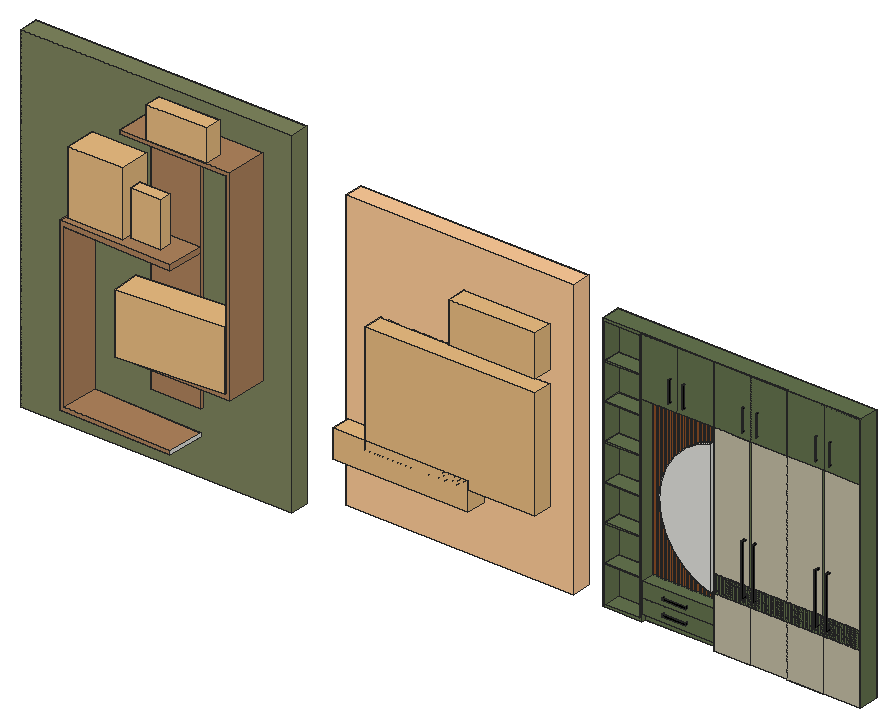
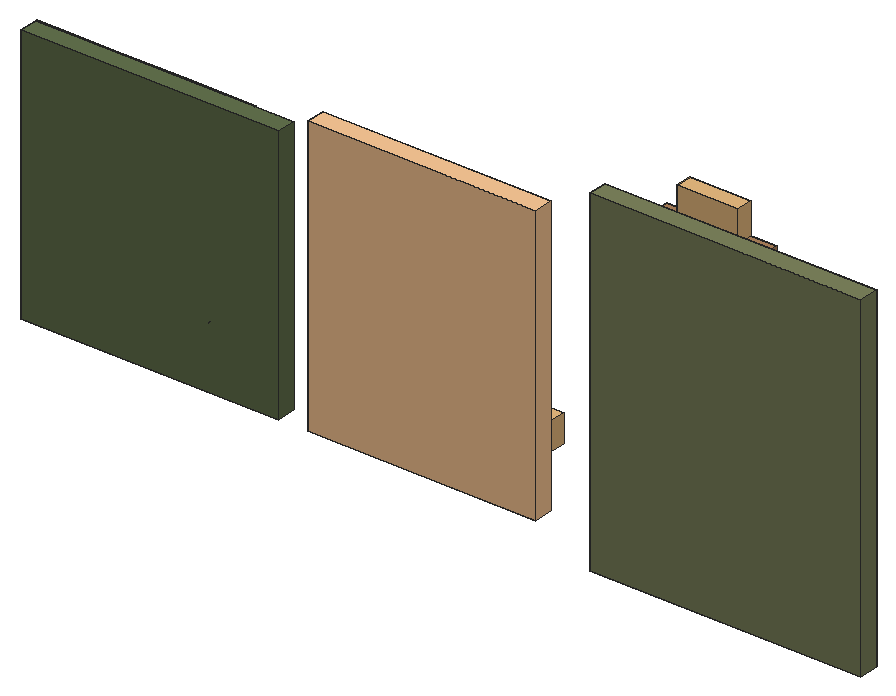
# SketchUp Ruby script. Lengths in inches.
U = 1.inch
M = Sketchup.active_model
def pt(a) = Geom::Point3d.new(a.map { |v| v * U })
def face(e, loops, mat)
  f = e.add_face(loops[0].map { |a| pt(a) })
  loops[1..].each { |l| e.add_face(l.map { |a| pt(a) }).erase! }
  f.material = f.back_material = mat if mat
  f
end
# faces: each face lists its corners as indices into pts; further lists are holes
def faces(e, pts, list, mat = nil) = list.each { |f| face(e, (f[0].is_a?(Array) ? f : [f]).map { |l| l.map { |i| pts[i] } }, mat) }
# xy, xz, yz: faces in a plane at the given z, y or x. An outline is a flat list of corners, or four numbers for a rectangle; further outlines are holes
def ring(l) = l.size == 4 ? [[l[0], l[1]], [l[2], l[1]], [l[2], l[3]], [l[0], l[3]]] : l.each_slice(2).to_a
def flat(e, list, mat, &to3) = list.each { |f| face(e, (f[0].is_a?(Array) ? f : [f]).map { |l| ring(l).map { |u, v| to3.(u, v) } }, mat) }
def xy(e, z, list, mat = nil) = flat(e, list, mat) { |x, y| [x, y, z] }
def xz(e, y, list, mat = nil) = flat(e, list, mat) { |x, z| [x, y, z] }
def yz(e, x, list, mat = nil) = flat(e, list, mat) { |y, z| [x, y, z] }
def lines(e, pts, list) = list.each { |a, b| e.add_line(pt(pts[a]), pt(pts[b])) }
# prism: a flat outline (further loops are holes) pulled along v
def prism(e, loops, v, mat = nil)
  f = face(e, loops, mat); d = Geom::Vector3d.new(v.map { |x| x * U })
  f.pushpull(f.normal.samedirection?(d) ? d.length : -d.length)
end
def box(e, o, s, mat = nil) = prism(e, [[o, [o[0] + s[0], o[1], o[2]], [o[0] + s[0], o[1] + s[1], o[2]], [o[0], o[1] + s[1], o[2]]]], [0, 0, s[2]], mat)
def at(x, y, z, deg = 0) = Geom::Transformation.translation(pt([x, y, z])) * Geom::Transformation.rotation(ORIGIN, Z_AXIS, deg.degrees)
def axes(o, x, y, z) = Geom::Transformation.new([*x, 0, *y, 0, *z, 0, *pt(o).to_a, 1])
def part(name) = M.definitions.add(name)
# library, detail: a bought-in or finely detailed component or shape, given as its bounding box
def library(name, o, s) = part(name).tap { |d| box(d.entities, o, s) }
def detail(e, o, s) = box(e.add_group.entities, o, s)
def put(e, d, t, mat = nil) = e.add_instance(d, t).tap { |i| i.material = mat if mat }
def group(e, t, mat = nil) = e.add_group.tap { |g| g.transformation = t; g.material = mat if mat }.entities
root = M.entities
M.materials.add("[Color A01]").color = [101, 116, 79]
M.materials.add("[Color A01]1").color = [196, 189, 165]
M.materials.add("[Color A01]2").color = [176, 132, 93]
M.materials.add("[Color A02]").color = [127, 133, 94]
M.materials.add("[Color C02]").color = [255, 204, 153]
M.materials.add("[Color M09]").color = [0, 0, 0]
M.materials.add("[Wood Cherry Original]").color = [152, 86, 42]
c1 = library("Untitled",[0,0,0],[7.78,10.125,9.38])
c2 = library("Ceramic Birds on",[-120.01,56.07,-27.09],[117.74,27.05,54.18])
c3 = library("SimLab\#1",[-237.64,52,0],[43.92,43.98,50.37])
c4 = part("Vertical wood slat")
box(c4.entities,[0,-2,0],[1,2,76],"[Wood Cherry Original]")
c5 = part("Group\#7")
prism(c5.entities,[[[0.625,2,0],[0.625,2,0.59],[0.625,0.59,0.59],[0.625,0.59,23.53],[0.625,2,23.53],[0.625,2,24.13],[0.625,0,24.13],[0.625,0,0]]],[-0.625,0,0])
c6 = part("Group\#5")
prism(c6.entities,[[[0.5,1,9.71],[0.5,1,10],[0.5,0,10],[0.5,0,0],[0.5,1,0],[0.5,1,0.29],[0.5,0.29,0.29],[0.5,0.29,9.71]]],[-0.5,0,0])
c7 = library("Group\#37",[208.35,-82.82,84.7],[13.92,5.45,20.99])
xy(root,5.8,[[84.22,0.51,32.41,1.51,32.74,19,84.56,18]],"[Color A01]2")
xy(root,84.7,[[84.22,0.51,84.56,18,32.74,19,32.41,1.51]],"[Color A01]2")
p = [[84.22,0.51,5.8],[84.22,0.51,7.18],[34.4,1.47,7.8],[34.4,1.47,82.7],[84.22,0.51,82.08],[84.22,0.51,84.7],
  [32.41,1.51,84.7],[32.41,1.51,5.8],[84.56,18,5.8],[84.56,18,7.18],[32.74,19,84.7],[32.74,19,5.8],
  [84.56,18,84.7],[84.56,18,82.08],[34.74,18.96,82.7],[34.74,18.96,7.8]]
faces(root,p,[[0,1,2,3,4,5,6,7],[10,11,7,6],[3,2,15,14],[4,3,14,13],[4,13,12,5]],"[Color A01]2")
faces(root,p,[[8,9,1,0],[12,13,14,15,9,8,11,10]])
put(root,c1,axes([110.34,0.03,40.32],[-0.12671,1.68524,0],[-4.76654,-0.3584,0],[0,0,3]))
put(root,c2,axes([102.2,-15.7,140.64],[0.23902,0,0],[0,0.28,0],[0,0,0.2698]))
put(root,c3,axes([171.33,-17.61,84.65],[0.58,0,0],[0,0.4272,0],[0,0,0.59]))
g1 = group(root,at(270.37,16.53,0))
prism(g1,[[[39.05,2.47,12.84],[39.35,2.47,12.84],[39.35,1.47,12.84],[28.35,1.47,12.84],[28.35,2.47,12.84],[28.65,2.47,12.84],[28.65,1.77,12.84],[39.05,1.77,12.84]]],[0,0,1],"[Color M09]")
prism(g1,[[[39.05,2.47,6],[39.35,2.47,6],[39.35,1.47,6],[28.35,1.47,6],[28.35,2.47,6],[28.65,2.47,6],[28.65,1.77,6],[39.05,1.77,6]]],[0,0,1],"[Color M09]")
put(g1,c4,at(34.23,10.47,17))
put(g1,c4,at(24.23,10.47,17))
put(g1,c4,at(46.23,10.47,17))
put(g1,c4,at(48.23,10.47,17))
put(g1,c4,at(44.23,10.47,17))
put(g1,c4,at(18.23,10.47,17))
put(g1,c4,at(20.23,10.47,17))
put(g1,c4,at(26.23,10.47,17))
put(g1,c4,at(42.23,10.47,17))
put(g1,c4,at(28.23,10.47,17))
put(g1,c4,at(36.23,10.47,17))
put(g1,c4,at(30.23,10.47,17))
put(g1,c4,at(22.23,10.47,17))
put(g1,c4,at(32.23,10.47,17))
put(g1,c4,at(38.23,10.47,17))
put(g1,c4,at(40.23,10.47,17))
put(g1,c4,at(50.23,10.47,17))
put(g1,c4,at(54.23,10.47,17))
put(g1,c4,at(58.23,10.47,17))
put(g1,c4,at(52.23,10.47,17))
put(g1,c4,at(56.23,10.47,17))
g2 = group(g1,at(23.23,8.39,20.33))
xz(g2,0,[[[24,0,17.44,2.49,11.58,6.35,6.7,11.4,3.04,17.38,0.77,24.02,0,31,0.77,37.98,3.04,44.62,6.7,50.6,11.58,55.65,17.44,59.51,24,62],[21.5,3.63,21.5,58.37,18.59,57.27,13.1875,53.71,8.69,49.06,5.32,43.54,3.23,37.43,2.52,31,3.23,24.57,5.32,18.46,8.69,12.94,13.1875,8.29,18.59,4.73]]])
g3 = group(g1,at(23.23,6.31,20.33))
xz(g3,0,[[24,0,24,62,17.44,59.51,11.58,55.65,6.7,50.6,3.04,44.62,0.77,37.98,0,31,0.77,24.02,3.04,17.38,6.7,11.4,11.58,6.35,17.44,2.49]])
xz(g3,2,[[[24,0,17.44,2.49,11.58,6.35,6.7,11.4,3.04,17.38,0.77,24.02,0,31,0.77,37.98,3.04,44.62,6.7,50.6,11.58,55.65,17.44,59.51,24,62],[21.5,3.63,21.5,58.37,18.59,57.27,13.1875,53.71,8.69,49.06,5.32,43.54,3.23,37.43,2.52,31,3.23,24.57,5.32,18.46,8.69,12.94,13.1875,8.29,18.59,4.73]],[21.5,3.63,18.59,4.73,13.1875,8.29,8.69,12.94,5.32,18.46,3.23,24.57,2.52,31,3.23,37.43,5.32,43.54,8.69,49.06,13.1875,53.71,18.59,57.27,21.5,58.37]])
yz(g3,24,[[0,0,2,62]])
p = [[24,0,0],[17.44,0,2.49],[17.44,2,2.49],[24,2,0],[11.58,0,6.35],[11.58,2,6.35],
  [6.7,0,11.4],[6.7,2,11.4],[3.04,0,17.38],[3.04,2,17.38],[0.77,0,24.02],[0.77,2,24.02],
  [0,0,31],[0,2,31],[0.77,0,37.98],[0.77,2,37.98],[3.04,0,44.62],[3.04,2,44.62],
  [6.7,0,50.6],[6.7,2,50.6],[11.58,0,55.65],[11.58,2,55.65],[17.44,0,59.51],[17.44,2,59.51],
  [24,0,62],[24,2,62]]
faces(g3,p,[[0,1,2,3],[1,4,5,2],[4,6,7,5],[6,8,9,7],[8,10,11,9],[10,12,13,11],[12,14,15,13],[14,16,17,15],
  [16,18,19,17],[18,20,21,19],[20,22,23,21],[22,24,25,23]])
g4 = group(g1,at(0,2.47,0),"[Color A01]")
xy(g4,0,[[52.232,-0.472,69.056,0],[69.295,-0.472,85.998,0],[86.234,-0.472,102.94,0],[103.176,-0.472,119.882,0],[0,0,0,9,120,9,120,0,52.232,0,52.232,8,18.232,8,18.232,0]])
xy(g4,1,[[1,0,17.232,8]])
xy(g4,17.857,[[1,0,17.232,8]])
xy(g4,18.357,[[1,0,17.232,8]])
xy(g4,34.714,[[1,0,17.232,8]])
xy(g4,35.214,[[1,0,17.232,8]])
xy(g4,51.571,[[1,0,17.232,8]])
xy(g4,52.071,[[1,0,17.232,8]])
xy(g4,68.429,[[1,0,17.232,8]])
xy(g4,68.929,[[1,0,17.232,8]])
xy(g4,85.286,[[1,0,17.232,8]])
xy(g4,85.786,[[1,0,17.232,8]])
xy(g4,93,[[18.232,-0.472,52.037,0],[52.232,-0.472,52.273,0],[52.273,-0.472,69.056,0],[69.056,-0.472,69.295,0],[69.295,-0.472,85.959,0],
  [85.959,-0.472,85.998,0],[86.196,-0.472,86.234,0],[86.234,-0.472,102.94,0],[102.94,-0.472,103.176,0],[103.176,-0.472,119.882,0],
  [119.882,-0.472,120,0],[18.232,0,52.037,8],[52.037,0,52.155,8],[52.155,0,52.232,8]])
xy(g4,102.143,[[1,0,17.232,8]])
xy(g4,102.643,[[1,0,17.232,8]])
xy(g4,119,[[1,0,17.232,8]])
xy(g4,120,[[18.232,-0.472,52.037,0],[52.273,-0.472,85.959,0],[86.196,-0.472,120,0],[0,0,120,9]])
xz(g4,-0.472,[[52.81,24,53.232,32],[53.81,24,54.232,32],[54.81,24,55.232,32],[55.81,24,56.232,32],[56.81,24,57.232,32],
  [57.81,24,58.232,32],[58.81,24,59.232,32],[59.81,24,60.232,32],[60.81,24,61.232,32],[61.81,24,62.232,32],
  [62.81,24,63.232,32],[63.81,24,64.232,32],[64.81,24,65.232,32],[65.81,24,66.232,32],[66.81,24,67.232,32],
  [67.81,24,68.232,32],[68.81,24,69.232,32],[69.81,24,70.232,32],[70.81,24,71.232,32],[71.81,24,72.232,32],
  [72.81,24,73.232,32],[73.81,24,74.232,32],[74.81,24,75.232,32],[75.81,24,76.232,32],[76.81,24,77.232,32],
  [77.81,24,78.232,32],[78.81,24,79.232,32],[79.81,24,80.232,32],[80.81,24,81.232,32],[81.81,24,82.232,32],
  [82.81,24,83.232,32],[83.81,24,84.232,32],[84.81,24,85.232,32],[85.81,24,86.232,32],[86.81,24,87.232,32],
  [87.81,24,88.232,32],[88.81,24,89.232,32],[89.81,24,90.232,32],[90.81,24,91.232,32],[91.81,24,92.232,32],
  [92.81,24,93.232,32],[93.81,24,94.232,32],[94.81,24,95.232,32],[95.81,24,96.232,32],[96.81,24,97.232,32],
  [97.81,24,98.232,32],[98.81,24,99.232,32],[99.81,24,100.232,32],[100.81,24,101.232,32],[101.81,24,102.232,32],
  [102.81,24,103.232,32],[103.81,24,104.232,32],[104.81,24,105.232,32],[105.81,24,106.232,32],[106.81,24,107.232,32],
  [107.81,24,108.232,32],[108.81,24,109.232,32],[109.81,24,110.232,32],[110.81,24,111.232,32],[111.81,24,112.232,32],
  [112.81,24,113.232,32],[113.81,24,114.232,32],[114.81,24,115.232,32],[115.81,24,116.232,32],[116.81,24,117.232,32],
  [117.81,24,118.232,32],[118.81,24,119.232,32],[119.81,24,119.882,32],[69.056,32,69.295,93],[102.94,32,103.176,93]])
xz(g4,-0.472,[[52.232,24,52.81,32],[53.232,24,53.81,32],[54.232,24,54.81,32],[55.232,24,55.81,32],[56.232,24,56.81,32],
  [57.232,24,57.81,32],[58.232,24,58.81,32],[59.232,24,59.81,32],[60.232,24,60.81,32],[61.232,24,61.81,32],
  [62.232,24,62.81,32],[63.232,24,63.81,32],[64.232,24,64.81,32],[65.232,24,65.81,32],[66.232,24,66.81,32],
  [67.232,24,67.81,32],[68.232,24,68.81,32],[69.232,24,69.81,32],[70.232,24,70.81,32],[71.232,24,71.81,32],
  [72.232,24,72.81,32],[73.232,24,73.81,32],[74.232,24,74.81,32],[75.232,24,75.81,32],[76.232,24,76.81,32],
  [77.232,24,77.81,32],[78.232,24,78.81,32],[79.232,24,79.81,32],[80.232,24,80.81,32],[81.232,24,81.81,32],
  [82.232,24,82.81,32],[83.232,24,83.81,32],[84.232,24,84.81,32],[85.232,24,85.81,32],[86.232,24,86.81,32],
  [87.232,24,87.81,32],[88.232,24,88.81,32],[89.232,24,89.81,32],[90.232,24,90.81,32],[91.232,24,91.81,32],
  [92.232,24,92.81,32],[93.232,24,93.81,32],[94.232,24,94.81,32],[95.232,24,95.81,32],[96.232,24,96.81,32],
  [97.232,24,97.81,32],[98.232,24,98.81,32],[99.232,24,99.81,32],[100.232,24,100.81,32],[101.232,24,101.81,32],
  [102.232,24,102.81,32],[103.232,24,103.81,32],[104.232,24,104.81,32],[105.232,24,105.81,32],[106.232,24,106.81,32],
  [107.232,24,107.81,32],[108.232,24,108.81,32],[109.232,24,109.81,32],[110.232,24,110.81,32],[111.232,24,111.81,32],
  [112.232,24,112.81,32],[113.232,24,113.81,32],[114.232,24,114.81,32],[115.232,24,115.81,32],[116.232,24,116.81,32],
  [117.232,24,117.81,32],[118.232,24,118.81,32],[119.232,24,119.81,32],[18.232,93,35.135,120],[35.135,93,52.037,120],
  [52.273,93,69.116,120],[69.116,93,85.959,120],[86.196,93,103.098,120],[103.098,93,120,120]],"[Color A01]")
xz(g4,-0.472,[[52.232,0,69.056,24],[69.295,0,85.998,24],[86.234,0,102.94,24],[103.176,0,119.882,24],[52.232,32,69.056,93],
  [69.295,32,85.998,93],[86.234,32,102.94,93],[103.176,32,119.882,93]],"[Color A01]1")
xz(g4,0,[[[0,0,18.232,120],[1,1,17.232,119]],[52.232,0,69.056,93],[69.056,0,69.174,93],[69.174,0,69.295,93],[69.295,0,85.998,93],
  [85.998,0,86.234,93],[86.234,0,102.94,93],[102.94,0,103.058,93],[103.058,0,103.176,93],[103.176,0,119.882,93],
  [119.882,0,120,93],[1,17.857,17.232,18.357],[1,34.714,17.232,35.214],[1,51.571,17.232,52.071],[1,68.429,17.232,68.929],
  [1,85.286,17.232,85.786],[18.232,93,52.037,120],[52.037,93,52.273,120],[52.273,93,85.959,120],[85.959,93,86.196,120],
  [86.196,93,120,120],[1,102.143,17.232,102.643]])
xz(g4,8,[[18.232,0,52.232,93],[1,1,17.232,18.357],[1,18.357,17.232,35.214],[1,35.214,17.232,52.071],[1,52.071,17.232,68.929],
  [1,68.929,17.232,85.786],[1,85.786,17.232,102.643],[1,102.643,17.232,119]])
xz(g4,9,[[0,0,120,120]])
yz(g4,0,[[0,0,9,120]])
yz(g4,1,[[0,1,8,18.357],[0,18.357,8,35.214],[0,35.214,8,52.071],[0,52.071,8,68.929],[0,68.929,8,85.786],
  [0,85.786,8,102.643],[0,102.643,8,119]])
yz(g4,17.232,[[0,1,8,18.357],[0,18.357,8,35.214],[0,35.214,8,52.071],[0,52.071,8,68.929],[0,68.929,8,85.786],
  [0,85.786,8,102.643],[0,102.643,8,119]])
yz(g4,18.232,[[0,0,8,93],[-0.472,93,0,120]])
yz(g4,52.037,[[-0.472,93,0,120]])
yz(g4,52.232,[[-0.472,0,0,93],[0,0,8,93]])
yz(g4,52.273,[[-0.472,93,0,120]])
yz(g4,85.959,[[-0.472,93,0,120]])
yz(g4,86.196,[[-0.472,93,0,120]])
yz(g4,119.882,[[-0.472,0,0,93]])
yz(g4,120,[[0,0,9,120],[-0.472,93,0,120]])
g5 = group(g1,at(18.23,2.47,0),"[Color A01]")
xy(g5,0,[[0,2,34,8]])
xy(g5,3,[[0,0,34,2],[0,2,34,8]])
xy(g5,10,[[0,0,34,8]])
xy(g5,17,[[0,0,34,8]])
xz(g5,0,[[0,3,34,10],[0,10,34,17]])
xz(g5,2,[[0,0,34,3]])
xz(g5,8,[[0,0,34,3],[0,3,34,10],[0,10,34,17]])
yz(g5,0,[[2,0,8,3],[0,3,8,10],[0,10,8,17]])
yz(g5,34,[[2,0,8,3],[0,3,8,10],[0,10,8,17]])
put(g1,c5,at(105.1875,0,27.21),"[Color M09]")
g6 = group(g1,at(66.1875,0,27.21),"[Color M09]")
prism(g6,[[[0.625,2,0],[0.625,2,0.59],[0.625,0.59,0.59],[0.625,0.59,23.53],[0.625,2,23.53],[0.625,2,24.13],[0.625,0,24.13],[0.625,0,0]]],[-0.625,0,0])
put(g1,c5,at(71.1875,0,27.21),"[Color M09]")
put(g1,c5,at(100.1875,0,27.21),"[Color M09]")
put(g1,c6,at(38.13,1,96),"[Color M09]")
put(g1,c6,at(65.68,1,96),"[Color M09]")
put(g1,c6,at(99.6,1,96),"[Color M09]")
put(g1,c6,at(72.18,1,96),"[Color M09]")
put(g1,c6,at(106.1,1,96),"[Color M09]")
put(g1,c6,at(31.63,1,96),"[Color M09]")
g7 = group(root,at(150.98,10,0))
detail(g7,[55.07,0,89.96],[40,9,19])
detail(g7,[16.27,0,32.91],[78.8,9,51.05])
detail(g7,[1.29,0,23.67],[63,9,12.92])
g8 = group(g7,at(0,9,6),"[Color C02]")
box(g8,[0,0,-6],[106,9,129])
g9 = group(root,at(0,19,0),"[Color A02]")
box(g9,[0,0,-12],[126,9,157])
g10 = group(root,at(61.56,0,38.33),"[Color A01]2")
prism(g10,[[[0,0,95],[0,0,93],[49,0,93],[49,0,2],[0,0,2],[0,0,0],[51,0,0],[51,0,95]]],[0,19,0])
g11 = group(root,at(61.56,18,17.33),"[Color A01]2")
box(g11,[0,0,0],[23,1,114])
g12 = group(root,at(34.4,0.51,7.18),"[Color A01]2")
p = [[0,0.96,0.62],[49.8125,0,0],[50.15,17.49,0],[0.34,18.45,0.62]]
faces(g12,p,[[0,1,2,3]])
put(root,c7,at(-147.63,89.93,0))
